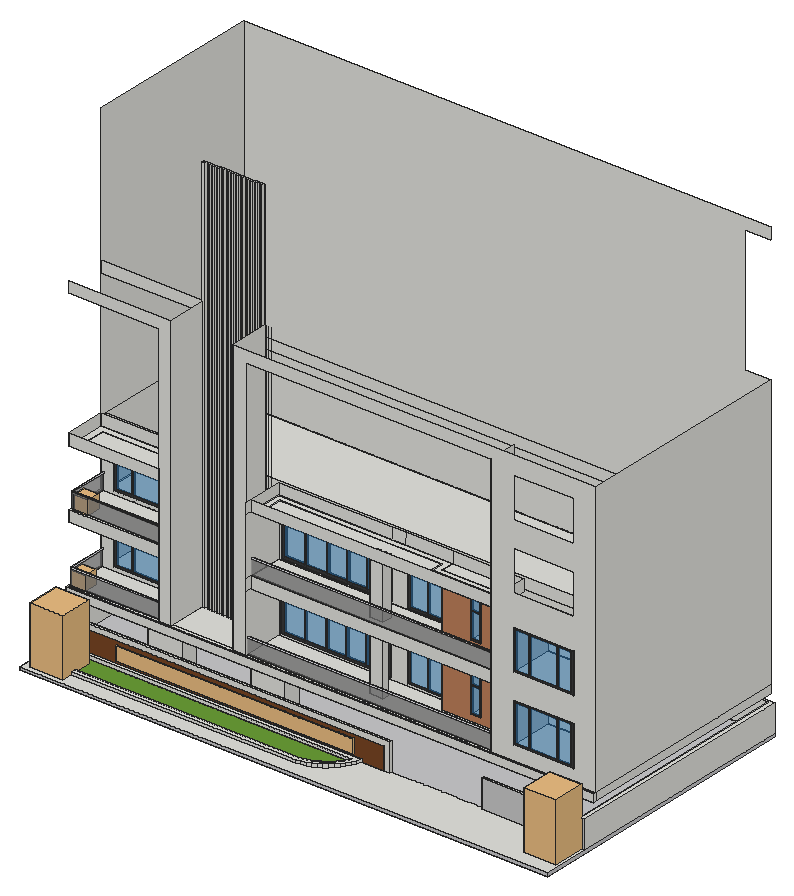
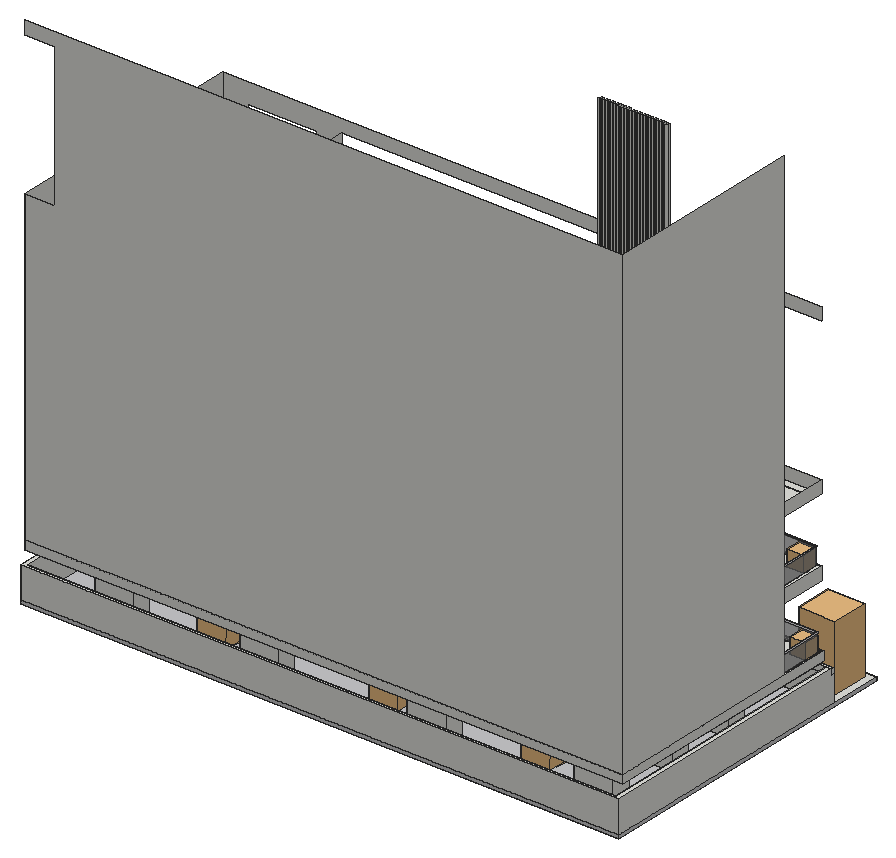
# SketchUp Ruby script. Lengths in inches.
U = 1.inch
M = Sketchup.active_model
def pt(a) = Geom::Point3d.new(a.map { |v| v * U })
def face(e, loops, mat)
  f = e.add_face(loops[0].map { |a| pt(a) })
  loops[1..].each { |l| e.add_face(l.map { |a| pt(a) }).erase! }
  f.material = f.back_material = mat if mat
  f
end
# faces: each face lists its corners as indices into pts; further lists are holes
def faces(e, pts, list, mat = nil) = list.each { |f| face(e, (f[0].is_a?(Array) ? f : [f]).map { |l| l.map { |i| pts[i] } }, mat) }
# xy, xz, yz: faces in a plane at the given z, y or x. An outline is a flat list of corners, or four numbers for a rectangle; further outlines are holes
def ring(l) = l.size == 4 ? [[l[0], l[1]], [l[2], l[1]], [l[2], l[3]], [l[0], l[3]]] : l.each_slice(2).to_a
def flat(e, list, mat, &to3) = list.each { |f| face(e, (f[0].is_a?(Array) ? f : [f]).map { |l| ring(l).map { |u, v| to3.(u, v) } }, mat) }
def xy(e, z, list, mat = nil) = flat(e, list, mat) { |x, y| [x, y, z] }
def xz(e, y, list, mat = nil) = flat(e, list, mat) { |x, z| [x, y, z] }
def yz(e, x, list, mat = nil) = flat(e, list, mat) { |y, z| [x, y, z] }
def lines(e, pts, list) = list.each { |a, b| e.add_line(pt(pts[a]), pt(pts[b])) }
# prism: a flat outline (further loops are holes) pulled along v
def prism(e, loops, v, mat = nil)
  f = face(e, loops, mat); d = Geom::Vector3d.new(v.map { |x| x * U })
  f.pushpull(f.normal.samedirection?(d) ? d.length : -d.length)
end
def box(e, o, s, mat = nil) = prism(e, [[o, [o[0] + s[0], o[1], o[2]], [o[0] + s[0], o[1] + s[1], o[2]], [o[0], o[1] + s[1], o[2]]]], [0, 0, s[2]], mat)
def at(x, y, z, deg = 0) = Geom::Transformation.translation(pt([x, y, z])) * Geom::Transformation.rotation(ORIGIN, Z_AXIS, deg.degrees)
def axes(o, x, y, z) = Geom::Transformation.new([*x, 0, *y, 0, *z, 0, *pt(o).to_a, 1])
def part(name) = M.definitions.add(name)
# library, detail: a bought-in or finely detailed component or shape, given as its bounding box
def library(name, o, s) = part(name).tap { |d| box(d.entities, o, s) }
def detail(e, o, s) = box(e.add_group.entities, o, s)
def put(e, d, t, mat = nil) = e.add_instance(d, t).tap { |i| i.material = mat if mat }
def group(e, t, mat = nil) = e.add_group.tap { |g| g.transformation = t; g.material = mat if mat }.entities
root = M.entities
M.materials.add("[Cladding Stucco White]").color = [200, 200, 200]
M.materials.add("[Color M00]").color = [255, 255, 255]
M.materials.add("[Color M07]").color = [58, 58, 58]
M.materials.add("[Grass Dark Green]").color = [106, 157, 55]
M.materials.add("[Metal Silver]").color = [234, 233, 238]
M.materials.add("[Polished Concrete New]").color = [200, 200, 203]
M.materials.add("[Translucent Glass Gray]").color = [40, 128, 199]
M.materials["[Translucent Glass Gray]"].alpha = 0.5
M.materials.add("[Translucent Glass Gray]1").color = [128, 128, 128]
M.materials["[Translucent Glass Gray]1"].alpha = 0.5
M.materials.add("[Wood Veneer 01]").color = [120, 70, 37]
M.materials.add("[Wood Veneer 02]").color = [190, 128, 91]
c1 = library("skp28\#1",[-2.51,-5.3125,0.36],[4.33,10.51,2.73])
c2 = part("ske164\#1")
put(c2.entities,c1,axes([101.27,98.68,1.14],[21.38,0,0],[0,21.38,0],[0,0,21.38]))
c3 = library("ske17D",[0,0,0],[82.9,31.14,82.9])
c4 = part("Sedan car")
put(c4.entities,c2,at(-47.7,14.91,-2.5))
put(c4.entities,c3,axes([87.34,31.1,0],[0,0.35842,0],[-0.35842,0,0],[0,0,0.35842]))
put(c4.entities,c3,axes([87.34,160.85,0],[0,0.35842,0],[-0.35842,0,0],[0,0,0.35842]))
put(c4.entities,c3,axes([5.18,190.5625,0],[0,-0.35842,0],[0.35842,0,0],[0,0,0.35842]))
put(c4.entities,c3,axes([5.43,60.8125,0],[0,-0.35842,0],[0.35842,0,0],[0,0,0.35842]))
c5 = part("Audi car")
put(c5.entities,c4,axes([116.24,65.71,-0.51],[0.88343,0,-0.01128],[0.00041,0.88291,0.03237],[0.01127,-0.03237,0.88283]))
c6 = library("trees",[-21.19,-21.7,-0.46],[44.22,41.02,72.81])
c7 = library("ROSELINE\#1",[1.48,0,0],[414.76,59.92,4])
c8 = library("plants",[-16.3,-15.81,0],[32.6,31.62,37.8])
c9 = part("Group\#3")
xy(c9.entities,0,[[0,0,103.1875,6]],"[Color M07]")
xy(c9.entities,6.75,[[6.75,0,49.1,6],[51.71,0,96.4375,6]],"[Color M07]")
xy(c9.entities,160.21,[[6.75,0,49.1,6],[51.71,0,96.4375,6]],"[Color M07]")
xy(c9.entities,166.96,[[0,0,103.1875,6]],"[Color M07]")
xz(c9.entities,0,[[[0,0,103.1875,166.96],[51.71,6.75,96.4375,160.21],[6.75,6.75,49.1,160.21]]],"[Color M07]")
xz(c9.entities,0,[[6.75,6.75,49.1,160.21],[51.71,6.75,96.4375,160.21]],"[Translucent Glass Gray]")
xz(c9.entities,6,[[[0,0,103.1875,166.96],[51.71,6.75,96.4375,160.21],[6.75,6.75,49.1,160.21]]],"[Color M07]")
yz(c9.entities,0,[[0,0,6,166.96]],"[Color M07]")
yz(c9.entities,6.75,[[0,6.75,6,160.21]],"[Color M07]")
yz(c9.entities,49.1,[[0,6.75,6,160.21]],"[Color M07]")
yz(c9.entities,51.71,[[0,6.75,6,160.21]],"[Color M07]")
yz(c9.entities,96.4375,[[0,6.75,6,160.21]],"[Color M07]")
yz(c9.entities,103.1875,[[0,0,6,166.96]],"[Color M07]")
c10 = part("Group\#2")
xy(c10.entities,0,[[0,0,266.875,6]],"[Color M07]")
xy(c10.entities,9.27,[[9.27,0,57.67,6],[61.37,0,109.48,6],[113.18,0,157.6,6],[161.3,0,205.85,6],[209.55,0,257.6,6]],"[Color M07]")
xy(c10.entities,155.66,[[9.27,0,57.67,6],[61.37,0,109.48,6],[113.18,0,157.6,6],[161.3,0,205.85,6],[209.55,0,257.6,6]],"[Color M07]")
xy(c10.entities,164.9375,[[0,0,266.875,6]],"[Color M07]")
xz(c10.entities,0,[[[0,0,266.875,164.9375],[9.27,9.27,57.67,155.66],[61.37,9.27,109.48,155.66],[209.55,9.27,257.6,155.66],[161.3,9.27,205.85,155.66],[113.18,9.27,157.6,155.66]]],"[Color M07]")
xz(c10.entities,0,[[9.27,9.27,57.67,155.66],[61.37,9.27,109.48,155.66],[113.18,9.27,157.6,155.66],[161.3,9.27,205.85,155.66],[209.55,9.27,257.6,155.66]],"[Translucent Glass Gray]")
xz(c10.entities,6,[[[0,0,266.875,164.9375],[9.27,9.27,57.67,155.66],[61.37,9.27,109.48,155.66],[209.55,9.27,257.6,155.66],[161.3,9.27,205.85,155.66],[113.18,9.27,157.6,155.66]]],"[Color M07]")
yz(c10.entities,0,[[0,0,6,164.9375]],"[Color M07]")
yz(c10.entities,9.27,[[0,9.27,6,155.66]],"[Color M07]")
yz(c10.entities,57.67,[[0,9.27,6,155.66]],"[Color M07]")
yz(c10.entities,61.37,[[0,9.27,6,155.66]],"[Color M07]")
yz(c10.entities,109.48,[[0,9.27,6,155.66]],"[Color M07]")
yz(c10.entities,113.18,[[0,9.27,6,155.66]],"[Color M07]")
yz(c10.entities,157.6,[[0,9.27,6,155.66]],"[Color M07]")
yz(c10.entities,161.3,[[0,9.27,6,155.66]],"[Color M07]")
yz(c10.entities,205.85,[[0,9.27,6,155.66]],"[Color M07]")
yz(c10.entities,209.55,[[0,9.27,6,155.66]],"[Color M07]")
yz(c10.entities,257.6,[[0,9.27,6,155.66]],"[Color M07]")
yz(c10.entities,266.875,[[0,0,6,164.9375]],"[Color M07]")
c11 = part("Group\#4")
xy(c11.entities,0,[[0,0,117.92,3.42]],"[Color M07]")
xy(c11.entities,5.06,[[5.06,0,29.89,3.42],[33.27,0,84.5,3.42],[87.88,0,112.86,3.42]],"[Color M07]")
xy(c11.entities,112.86,[[5.06,0,29.89,3.42],[33.27,0,84.5,3.42],[87.88,0,112.86,3.42]],"[Color M07]")
xy(c11.entities,117.92,[[0,0,117.92,3.42]],"[Color M07]")
xz(c11.entities,0,[[[0,0,117.92,117.92],[33.27,5.06,84.5,112.86],[87.88,5.06,112.86,112.86],[5.06,5.06,29.89,112.86]]],"[Color M07]")
xz(c11.entities,0,[[5.06,5.06,29.89,112.86],[33.27,5.06,84.5,112.86],[87.88,5.06,112.86,112.86]],"[Translucent Glass Gray]")
xz(c11.entities,3.42,[[[0,0,117.92,117.92],[33.27,5.06,84.5,112.86],[87.88,5.06,112.86,112.86],[5.06,5.06,29.89,112.86]]],"[Color M07]")
yz(c11.entities,0,[[0,0,3.42,117.92]],"[Color M07]")
yz(c11.entities,5.06,[[0,5.06,3.42,112.86]],"[Color M07]")
yz(c11.entities,29.89,[[0,5.06,3.42,112.86]],"[Color M07]")
yz(c11.entities,33.27,[[0,5.06,3.42,112.86]],"[Color M07]")
yz(c11.entities,84.5,[[0,5.06,3.42,112.86]],"[Color M07]")
yz(c11.entities,87.88,[[0,5.06,3.42,112.86]],"[Color M07]")
yz(c11.entities,112.86,[[0,5.06,3.42,112.86]],"[Color M07]")
yz(c11.entities,117.92,[[0,0,3.42,117.92]],"[Color M07]")
c12 = part("Group\#5")
xy(c12.entities,0,[[0,0,33.625,2.4375]],"[Color M07]")
xy(c12.entities,2.77,[[2.77,0,30.85,2.4375]],"[Color M07]")
xy(c12.entities,92.73,[[2.77,0,30.85,2.4375]],"[Color M07]")
xy(c12.entities,95.66,[[2.77,0,30.85,2.4375]],"[Color M07]")
xy(c12.entities,164.1,[[2.77,0,30.85,2.4375]],"[Color M07]")
xy(c12.entities,166.875,[[0,0,33.625,2.4375]],"[Color M07]")
xz(c12.entities,0,[[[0,0,33.625,166.875],[2.77,2.77,30.85,92.73],[2.77,95.66,30.85,164.1]]],"[Color M07]")
xz(c12.entities,0,[[2.77,2.77,30.85,92.73],[2.77,95.66,30.85,164.1]],"[Translucent Glass Gray]")
xz(c12.entities,2.4375,[[[0,0,33.625,166.875],[2.77,2.77,30.85,92.73],[2.77,95.66,30.85,164.1]]],"[Color M07]")
yz(c12.entities,0,[[0,0,2.4375,166.875]],"[Color M07]")
yz(c12.entities,2.77,[[0,2.77,2.4375,92.73],[0,95.66,2.4375,164.1]],"[Color M07]")
yz(c12.entities,30.85,[[0,2.77,2.4375,92.73],[0,95.66,2.4375,164.1]],"[Color M07]")
yz(c12.entities,33.625,[[0,0,2.4375,166.875]],"[Color M07]")
xy(root,0,[[0,0,1665.48,897.1]])
xy(root,9,[[0,0,1665.48,0,1665.48,149.5,1338.12,149.5,1338.12,157.51,1048.18,157.51,1048.18,149.5,958.59,149.5,953.98,136.02,948.06,123.06,940.88,110.75,932.53,99.2,923.07,88.54,912.61,78.87,901.25,70.28,889.09,62.85,876.25,56.66,862.87,51.77,849.07,48.23,834.98,46.0625,84.59,46.0625,84.59,149.5,0,149.5],[[84.59,46.0625,84.59,149.5,958.59,149.5,953.98,136.02,948.06,123.06,940.88,110.75,932.53,99.2,923.07,88.54,912.61,78.87,901.25,70.28,889.09,62.85,876.25,56.66,862.87,51.77,849.07,48.23,834.98,46.0625],[97.76,59.23,833.98,59.23,846.42,61.14,858.96,64.36,871.12,68.8,882.78,74.43,893.83,81.17,904.15,88.98,913.66,97.77,922.25,107.45,929.84,117.9375,936.35,129.12,939.65,136.33,97.76,136.33]],[0,149.5,0,897.1,1665.48,897.1,1665.48,149.5,1338.12,149.5,1338.12,157.51,1651.6,157.51,1651.6,889.09,13.88,889.09,13.88,157.51,1030.62,157.51,1030.62,149.5],[1030.62,149.5,1048.18,157.51],[221.91,227.7,330.82,281.1],
  [546.04,227.7,654.95,281.1],[81.13,358.18,190.04,411.58],[1412.71,362.14,1521.62,415.54],[81.13,553.59,190.04,606.99],[1412.71,567.51,1521.62,620.91],
  [81.13,760.57,190.04,813.97],[542.67,764.37,651.58,817.77],[1009.74,764.37,1118.65,817.77],[1412.71,764.37,1521.62,817.77]])
xy(root,9,[[97.76,59.23,833.98,59.23,846.42,61.14,858.96,64.36,871.12,68.8,882.78,74.43,893.83,81.17,904.15,88.98,913.66,97.77,922.25,107.45,929.84,117.9375,936.35,129.12,939.65,136.33,97.76,136.33]],"[Grass Dark Green]")
xy(root,9,[[[13.88,157.51,1651.6,889.09],[221.91,227.7,330.82,281.1],[546.04,227.7,654.95,281.1],[81.13,760.57,190.04,813.97],[81.13,553.59,190.04,606.99],[81.13,358.18,190.04,411.58],[1009.74,764.37,1118.65,817.77],[1412.71,764.37,1521.62,817.77],[1412.71,567.51,1521.62,620.91],[1412.71,362.14,1521.62,415.54],[542.67,764.37,651.58,817.77]]],"[Polished Concrete New]")
xy(root,17.8125,[[[84.59,46.0625,834.98,46.0625,849.07,48.23,862.87,51.77,876.25,56.66,889.09,62.85,901.25,70.28,912.61,78.87,923.07,88.54,932.53,99.2,940.88,110.75,948.06,123.06,953.98,136.02,958.59,149.5,84.59,149.5],[97.76,59.23,97.76,136.33,939.65,136.33,936.35,129.12,929.84,117.9375,922.25,107.45,913.66,97.77,904.15,88.98,893.83,81.17,882.78,74.43,871.12,68.8,858.96,64.36,846.42,61.14,833.98,59.23]]])
xy(root,98.25,[[0,149.5,1048.18,157.51],[1338.12,149.5,1665.48,149.5,1665.48,897.1,0,897.1,0,157.51,13.88,157.51,13.88,889.09,1651.6,889.09,1651.6,157.51,1338.12,157.51]])
xy(root,129,[[0,182.16,1665.48,191.16]])
xy(root,129,[[[0,191.16,1665.48,882.45],[221.91,227.7,330.82,281.1],[546.04,227.7,654.95,281.1],[1009.74,764.37,1118.65,817.77],[81.13,760.57,190.04,813.97],[1412.71,362.14,1521.62,415.54],[1412.71,567.51,1521.62,620.91],[542.67,764.37,651.58,817.77],[81.13,553.59,190.04,606.99],[81.13,358.18,190.04,411.58],[1412.71,764.37,1521.62,817.77]],[221.91,227.7,330.82,281.1],[546.04,227.7,654.95,281.1],[81.13,358.18,190.04,411.58],[1412.71,362.14,1521.62,415.54],
  [81.13,553.59,190.04,606.99],[1412.71,567.51,1521.62,620.91],[81.13,760.57,190.04,813.97],[542.67,764.37,651.58,817.77],[1009.74,764.37,1118.65,817.77],
  [1412.71,764.37,1521.62,817.77]],"[Color M00]")
xy(root,153,[[0,182.16,1665.48,182.16,1665.48,187.35,4.5625,187.35,4.5625,320.73,0,320.73],[4.5625,187.35,1665.48,187.35,1665.48,191.16,1334.26,191.16,1334.26,195.98,559.99,195.98,559.99,191.16,518.01,191.16,518.01,196.41,324.77,196.41,324.77,191.16,284.54,191.16,284.54,196.41,4.5625,196.41],[518.01,191.16,518.01,320.73,0,320.73,0,882.45,1561.7,882.45,1561.7,873.45,9.75,873.45,9.75,328.54,1561.7,328.54,1561.7,191.16,1334.26,191.16,1334.26,280.1,1109.39,280.1,1109.39,320.73,559.99,320.73,559.99,191.16],[284.54,191.16,324.77,320.73],[1561.7,191.16,1561.7,328.54,1655.73,328.54,1655.73,873.45,1561.7,873.45,1561.7,882.45,1665.48,882.45,1665.48,191.16],
  [559.99,195.98,1334.26,197.98],[4.5625,196.41,284.54,198.73],[[559.99,197.98,1334.26,197.98,1334.26,280.1,1109.39,280.1,1109.39,320.73,559.99,320.73],[917.6,233.32,960.55,250.32]],[4.5625,198.73,6.5625,320.73],[6.5625,198.73,284.54,320.73],
  [324.77,198.73,518.01,198.73,518.01,320.73,514,320.73,514,313.48,506.5,313.48,506.5,320.73,499,320.73,499,313.48,491.5,313.48,491.5,320.73,484,320.73,484,313.48,476.5,313.48,476.5,320.73,469,320.73,469,313.48,461.5,313.48,461.5,320.73,454,320.73,454,313.48,446.5,313.48,446.5,320.73,439,320.73,439,313.48,431.5,313.48,431.5,320.73,424,320.73,424,313.48,416.5,313.48,416.5,320.73,409,320.73,409,313.48,401.5,313.48,401.5,320.73,394,320.73,394,313.48,386.5,313.48,386.5,320.73,379,320.73,379,313.48,371.5,313.48,371.5,320.73,364,320.73,364,313.48,356.5,313.48,356.5,320.73,349,320.73,349,313.48,341.5,313.48,341.5,320.73,334,320.73,334,313.48,324.77,313.48],[917.6,233.32,960.55,250.32],[324.77,313.48,334,320.73],[341.5,313.48,349,320.73],[356.5,313.48,364,320.73],
  [371.5,313.48,379,320.73],[386.5,313.48,394,320.73],[401.5,313.48,409,320.73],[416.5,313.48,424,320.73],[431.5,313.48,439,320.73],
  [446.5,313.48,454,320.73],[461.5,313.48,469,320.73],[476.5,313.48,484,320.73],[491.5,313.48,499,320.73],[506.5,313.48,514,320.73],
  [9.75,328.54,1561.7,873.45],[1561.7,328.54,1655.73,873.45]])
xy(root,157.44,[[967.92,320.73,1101.04,328.54]])
xy(root,157.96,[[566.1875,320.73,914.8125,328.54]])
xy(root,163.04,[[40.45,320.73,260.7,328.54]])
xy(root,172.9,[[1200.375,280.1,1230.875,328.54]])
xy(root,196.42,[[1405.04,191.16,1595.91,328.54]])
xy(root,201,[[559.99,195.98,1334.26,197.98],[4.5625,196.41,4.5625,320.73,6.5625,320.73,6.5625,198.73,284.54,198.73,284.54,196.41]],"[Metal Silver]")
xy(root,205,[[559.99,195.98,1334.26,197.98],[4.5625,196.41,284.54,196.41,284.54,198.73,6.5625,198.73,6.5625,320.73,4.5625,320.73]],"[Metal Silver]")
xy(root,302.7,[[566.1875,320.73,914.8125,328.54],[967.92,320.73,1101.04,328.54]])
xy(root,316.92,[[40.45,320.73,260.7,328.54]])
xy(root,319.08,[[1200.375,280.1,1230.875,328.54]])
xy(root,324.73,[[1405.04,191.16,1595.91,328.54]])
xy(root,325,[[[578.25,228.93,578.25,302.47,1091.125,302.47,1091.125,261.84,1316,261.84,1316,228.93],[917.6,233.32,960.55,250.32]]])
xy(root,328,[[17.43,208.59,267.11,303.3]])
xy(root,333,[[[0,191.16,284.54,320.73],[17.43,208.59,267.11,303.3]],[17.43,208.59,267.11,303.3],[[559.99,210.66,559.99,320.73,1109.39,320.73,1109.39,280.1,1334.26,280.1,1334.26,210.66],[578.25,228.93,1316,228.93,1316,261.84,1091.125,261.84,1091.125,302.47,578.25,302.47]],[[578.25,228.93,1316,228.93,1316,261.84,1091.125,261.84,1091.125,302.47,578.25,302.47],[917.6,233.32,960.55,250.32]],[917.6,233.32,960.55,250.32],
  [1109.39,280.1,1334.26,320.73]])
xy(root,369,[[0,191.16,284.54,191.16,284.54,197.23,6.5625,197.23,6.5625,320.73,0,320.73],[6.5625,197.23,6.5625,320.73,8.5625,320.73,8.5625,199.23,284.54,199.23,284.54,197.23],[8.5625,199.23,284.54,320.73],[559.99,210.66,1334.26,212.66],[559.99,212.66,1334.26,214.66],
  [[559.99,214.66,1334.26,214.66,1334.26,280.1,1109.39,280.1,1109.39,320.73,559.99,320.73],[917.6,233.32,960.55,264.07]],[917.6,233.32,960.55,264.07],[1109.39,280.1,1334.26,320.73],[9.75,328.54,1561.7,873.45]])
xy(root,371.75,[[967.92,320.73,1101.04,328.54]])
xy(root,373.36,[[568.97,320.73,917.6,328.54]])
xy(root,379.67,[[40.45,320.73,260.7,328.54]])
xy(root,383.4,[[1200.375,280.1,1230.875,328.54]])
xy(root,402.17,[[1405.04,191.16,1595.91,328.54]])
xy(root,417,[[6.5625,197.23,6.5625,320.73,8.5625,320.73,8.5625,199.23,284.54,199.23,284.54,197.23],[559.99,212.66,1334.26,214.66]],"[Metal Silver]")
xy(root,421,[[6.5625,197.23,284.54,197.23,284.54,199.23,8.5625,199.23,8.5625,320.73,6.5625,320.73],[559.99,212.66,1334.26,214.66]],"[Metal Silver]")
xy(root,522.07,[[568.97,320.73,917.6,328.54],[967.92,320.73,1101.04,328.54]])
xy(root,529.58,[[1200.375,280.1,1230.875,328.54]])
xy(root,530.48,[[1405.04,191.16,1595.91,328.54]])
xy(root,533.54,[[40.45,320.73,260.7,328.54]])
xy(root,541,[[[578.25,228.93,578.25,302.47,1091.125,302.47,1091.125,261.84,1316,261.84,1316,228.93],[917.6,233.32,960.55,264.07]]])
xy(root,544,[[21.22,212.38,263.32,299.51]])
xy(root,549,[[[0,191.16,284.54,320.73],[21.22,212.38,263.32,299.51]],[[559.99,210.66,559.99,320.73,1109.39,320.73,1109.39,280.1,1334.26,280.1,1334.26,210.66],[578.25,228.93,1316,228.93,1316,261.84,1091.125,261.84,1091.125,302.47,578.25,302.47]],[21.22,212.38,263.32,299.51],[[578.25,228.93,1316,228.93,1316,261.84,1091.125,261.84,1091.125,302.47,578.25,302.47],[917.6,233.32,960.55,264.07]],[1109.39,280.1,1334.26,320.73]])
xz(root,0,[[0,0,1665.48,9]],"[Polished Concrete New]")
xz(root,46.0625,[[84.59,9,834.98,17.8125]])
xz(root,59.23,[[97.76,9,833.98,17.8125]])
xz(root,136.33,[[97.76,9,939.65,17.8125]])
xz(root,149.5,[[0,9,27.05,9,27.05,81,1030.62,81,1030.62,9,1048.18,9,1048.18,98.25,0,98.25],[84.59,9,958.59,17.8125]])
xz(root,149.5,[[1338.12,9,1665.48,98.25]],"[Cladding Stucco White]")
xz(root,149.5,[[27.05,9,84.59,9,84.59,17.8125,958.59,17.8125,958.59,9,1030.62,9,1030.62,81,27.05,81]],"[Wood Veneer 01]")
xz(root,157.51,[[1030.62,9,1030.62,81,13.88,81,13.88,98.25,1048.18,98.25,1048.18,9],[13.88,9,1030.62,81],[1338.12,9,1651.6,98.25]])
xz(root,182.16,[[0,129,1665.48,153]])
xz(root,191.16,[[284.54,153,324.77,153,324.77,1017,0,1017,0,981,284.54,981],[[518.01,153,559.99,153,559.99,981,1334.26,981,1334.26,153,1665.48,153,1665.48,1017,518.01,1017],[1405.04,832.73,1595.91,961.04],[1405.04,625.17,1595.91,753.48],[1405.04,196.42,1595.91,324.73],[1405.04,402.17,1595.91,530.48]],[0,333,284.54,369],[0,549,284.54,585]])
xz(root,195.98,[[559.99,201,1334.26,205]],"[Metal Silver]")
xz(root,195.98,[[559.99,153,1334.26,201]],"[Translucent Glass Gray]1")
xz(root,196.41,[[4.5625,201,284.54,205]],"[Metal Silver]")
xz(root,196.41,[[4.5625,153,284.54,201]],"[Translucent Glass Gray]1")
xz(root,197.23,[[6.5625,417,284.54,421]],"[Metal Silver]")
xz(root,197.23,[[6.5625,369,284.54,417]],"[Translucent Glass Gray]1")
xz(root,197.98,[[559.99,201,1334.26,205]],"[Metal Silver]")
xz(root,197.98,[[559.99,153,1334.26,201]],"[Translucent Glass Gray]1")
xz(root,198.73,[[6.5625,201,284.54,205]],"[Metal Silver]")
xz(root,198.73,[[6.5625,153,284.54,201]],"[Translucent Glass Gray]1")
xz(root,199.23,[[8.5625,417,284.54,421]],"[Metal Silver]")
xz(root,199.23,[[8.5625,369,284.54,417]],"[Translucent Glass Gray]1")
xz(root,208.59,[[17.43,328,267.11,333]])
xz(root,210.66,[[559.99,333,1334.26,369],[559.99,549,1334.26,585]])
xz(root,212.38,[[21.22,544,263.32,549]])
xz(root,212.66,[[559.99,417,1334.26,421]],"[Metal Silver]")
xz(root,212.66,[[559.99,369,1334.26,417]],"[Translucent Glass Gray]1")
xz(root,214.66,[[559.99,417,1334.26,421]],"[Metal Silver]")
xz(root,214.66,[[559.99,369,1334.26,417]],"[Translucent Glass Gray]1")
xz(root,227.7,[[221.91,9,330.82,129],[546.04,9,654.95,129]])
xz(root,228.93,[[578.25,325,1316,333],[578.25,541,1316,549]])
xz(root,233.32,[[917.6,153,960.55,325],[917.6,325,960.55,333],[917.6,369,960.55,541],[917.6,541,960.55,549]])
xz(root,250.32,[[917.6,153,960.55,325],[917.6,325,960.55,333]])
xz(root,261.84,[[1091.125,325,1316,333],[1091.125,541,1316,549]])
xz(root,264.07,[[917.6,369,960.55,541],[917.6,541,960.55,549]])
xz(root,280.1,[[[1109.39,153,1334.26,333],[1200.375,172.9,1230.875,319.08]],[[1109.39,369,1334.26,549],[1200.375,383.4,1230.875,529.58]]],"[Wood Veneer 02]")
xz(root,281.1,[[221.91,9,330.82,129],[546.04,9,654.95,129]])
xz(root,299.51,[[21.22,544,263.32,549]])
xz(root,302.47,[[578.25,325,917.6,333],[917.6,325,960.55,333],[960.55,325,1091.125,333],[578.25,541,917.6,549],[917.6,541,960.55,549],
  [960.55,541,1091.125,549]])
xz(root,303.3,[[17.43,328,267.11,333]])
xz(root,313.48,[[324.77,153,334,1413],[341.5,153,349,1413],[356.5,153,364,1413],[371.5,153,379,1413],[386.5,153,394,1413],
  [401.5,153,409,1413],[416.5,153,424,1413],[431.5,153,439,1413],[446.5,153,454,1413],[461.5,153,469,1413],
  [476.5,153,484,1413],[491.5,153,499,1413],[506.5,153,514,1413]])
xz(root,320.73,[[284.54,153,284.54,981,0,981,0,1017,324.77,1017,324.77,153],[[0,153,4.5625,153,4.5625,205,6.5625,205,6.5625,153,284.54,153,284.54,333,0,333],[40.45,163.04,260.7,316.92]],[4.5625,153,6.5625,201],[324.77,153,334,1413],[334,153,341.5,1413],
  [341.5,153,349,1413],[349,153,356.5,1413],[356.5,153,364,1413],[364,153,371.5,1413],[371.5,153,379,1413],
  [379,153,386.5,1413],[386.5,153,394,1413],[394,153,401.5,1413],[401.5,153,409,1413],[409,153,416.5,1413],
  [416.5,153,424,1413],[424,153,431.5,1413],[431.5,153,439,1413],[439,153,446.5,1413],[446.5,153,454,1413],
  [454,153,461.5,1413],[461.5,153,469,1413],[469,153,476.5,1413],[476.5,153,484,1413],[484,153,491.5,1413],
  [491.5,153,499,1413],[499,153,506.5,1413],[506.5,153,514,1413],[514,153,518.01,1413],[[559.99,153,1109.39,333],[566.1875,157.96,914.8125,302.7],[967.92,157.44,1101.04,302.7]],
  [0,333,284.54,369],[559.99,333,917.6,369],[917.6,333,960.55,369],[960.55,333,1109.39,369],[1109.39,333,1334.26,369],
  [[0,369,6.5625,369,6.5625,421,8.5625,421,8.5625,369,284.54,369,284.54,549,0,549],[40.45,379.67,260.7,533.54]],[6.5625,369,8.5625,417],[[559.99,369,1109.39,549],[568.97,373.36,917.6,522.07],[967.92,371.75,1101.04,522.07]],[0,549,284.54,585],[559.99,549,917.6,585],
  [917.6,549,960.55,585],[960.55,549,1109.39,585],[1109.39,549,1334.26,585]])
xz(root,320.73,[[4.5625,201,6.5625,205],[6.5625,417,8.5625,421]],"[Metal Silver]")
xz(root,328.54,[[[9.75,153,1655.73,333],[566.1875,157.96,914.8125,302.7],[40.45,163.04,260.7,316.92],[1405.04,196.42,1595.91,324.73],[967.92,157.44,1101.04,302.7],[1200.375,172.9,1230.875,319.08]],[9.75,333,1655.73,369],[[9.75,369,1655.73,549],[568.97,373.36,917.6,522.07],[40.45,379.67,260.7,533.54],[1405.04,402.17,1595.91,530.48],[967.92,371.75,1101.04,522.07],[1200.375,383.4,1230.875,529.58]],[9.75,549,1655.73,585]])
xz(root,358.18,[[81.13,9,190.04,129]])
xz(root,362.14,[[1412.71,9,1521.62,129]])
xz(root,411.58,[[81.13,9,190.04,129]])
xz(root,415.54,[[1412.71,9,1521.62,129]])
xz(root,553.59,[[81.13,9,190.04,129]])
xz(root,567.51,[[1412.71,9,1521.62,129]])
xz(root,606.99,[[81.13,9,190.04,129]])
xz(root,620.91,[[1412.71,9,1521.62,129]])
xz(root,760.57,[[81.13,9,190.04,129]])
xz(root,764.37,[[542.67,9,651.58,129],[1009.74,9,1118.65,129],[1412.71,9,1521.62,129]])
xz(root,813.97,[[81.13,9,190.04,129]])
xz(root,817.77,[[542.67,9,651.58,129],[1009.74,9,1118.65,129],[1412.71,9,1521.62,129]])
xz(root,873.45,[[9.75,153,1655.73,333],[9.75,333,1655.73,369],[9.75,369,1655.73,549],[9.75,549,1655.73,585]])
xz(root,882.45,[[0,129,1665.48,153],[0,153,0,1449,1665.48,1449,1665.48,1413,1581.35,1413,1581.35,1017,1665.48,1017,1665.48,153]])
xz(root,889.09,[[13.88,9,1651.6,98.25]])
xz(root,897.1,[[0,9,1665.48,98.25]])
xz(root,897.1,[[0,0,1665.48,9]],"[Polished Concrete New]")
yz(root,0,[[149.5,9,149.5,81,157.51,81,157.51,98.25,897.1,98.25,897.1,9],[149.5,81,157.51,98.25],[182.16,129,882.45,153],[320.73,153,882.45,1449],[191.16,333,320.73,369],
  [191.16,549,320.73,585]])
yz(root,0,[[0,0,897.1,9]],"[Polished Concrete New]")
yz(root,4.5625,[[196.41,201,320.73,205]],"[Metal Silver]")
yz(root,4.5625,[[196.41,153,320.73,201]],"[Translucent Glass Gray]1")
yz(root,6.5625,[[198.73,201,320.73,205],[197.23,417,320.73,421]],"[Metal Silver]")
yz(root,6.5625,[[198.73,153,320.73,201],[197.23,369,320.73,417]],"[Translucent Glass Gray]1")
yz(root,8.5625,[[199.23,417,320.73,421]],"[Metal Silver]")
yz(root,8.5625,[[199.23,369,320.73,417]],"[Translucent Glass Gray]1")
yz(root,9.75,[[328.54,153,873.45,369],[328.54,369,873.45,585]])
yz(root,13.88,[[157.51,9,889.09,98.25]])
yz(root,17.43,[[208.59,328,303.3,333]])
yz(root,21.22,[[212.38,544,299.51,549]])
yz(root,40.45,[[320.73,163.04,328.54,316.92],[320.73,379.67,328.54,533.54]])
yz(root,81.13,[[358.18,9,411.58,129],[553.59,9,606.99,129],[760.57,9,813.97,129]])
yz(root,84.59,[[46.0625,9,149.5,17.8125]])
yz(root,97.76,[[59.23,9,136.33,17.8125]])
yz(root,190.04,[[358.18,9,411.58,129],[553.59,9,606.99,129],[760.57,9,813.97,129]])
yz(root,221.91,[[227.7,9,281.1,129]])
yz(root,260.7,[[320.73,163.04,328.54,316.92],[320.73,379.67,328.54,533.54]])
yz(root,263.32,[[212.38,544,299.51,549]])
yz(root,267.11,[[208.59,328,303.3,333]])
yz(root,284.54,[[191.16,153,191.16,333,320.73,333,320.73,153,198.73,153,198.73,205,196.41,205,196.41,153],[196.41,153,198.73,201],[191.16,333,320.73,369],[191.16,369,191.16,549,320.73,549,320.73,369,199.23,369,199.23,421,197.23,421,197.23,369],[197.23,369,199.23,417],
  [191.16,549,320.73,585]])
yz(root,284.54,[[196.41,201,198.73,205],[197.23,417,199.23,421]],"[Metal Silver]")
yz(root,324.77,[[191.16,153,313.48,1017],[313.48,153,320.73,333],[313.48,333,320.73,369],[313.48,369,320.73,549],[313.48,549,320.73,585]])
yz(root,330.82,[[227.7,9,281.1,129]])
yz(root,334,[[313.48,153,320.73,1413]])
yz(root,341.5,[[313.48,153,320.73,1413]])
yz(root,349,[[313.48,153,320.73,1413]])
yz(root,356.5,[[313.48,153,320.73,1413]])
yz(root,364,[[313.48,153,320.73,1413]])
yz(root,371.5,[[313.48,153,320.73,1413]])
yz(root,379,[[313.48,153,320.73,1413]])
yz(root,386.5,[[313.48,153,320.73,1413]])
yz(root,394,[[313.48,153,320.73,1413]])
yz(root,401.5,[[313.48,153,320.73,1413]])
yz(root,409,[[313.48,153,320.73,1413]])
yz(root,416.5,[[313.48,153,320.73,1413]])
yz(root,424,[[313.48,153,320.73,1413]])
yz(root,431.5,[[313.48,153,320.73,1413]])
yz(root,439,[[313.48,153,320.73,1413]])
yz(root,446.5,[[313.48,153,320.73,1413]])
yz(root,454,[[313.48,153,320.73,1413]])
yz(root,461.5,[[313.48,153,320.73,1413]])
yz(root,469,[[313.48,153,320.73,1413]])
yz(root,476.5,[[313.48,153,320.73,1413]])
yz(root,484,[[313.48,153,320.73,1413]])
yz(root,491.5,[[313.48,153,320.73,1413]])
yz(root,499,[[313.48,153,320.73,1413]])
yz(root,506.5,[[313.48,153,320.73,1413]])
yz(root,514,[[313.48,153,320.73,1413]])
yz(root,518.01,[[191.16,153,320.73,1017]])
yz(root,542.67,[[764.37,9,817.77,129]])
yz(root,546.04,[[227.7,9,281.1,129]])
yz(root,559.99,[[191.16,153,195.98,153,195.98,205,197.98,205,197.98,153,320.73,153,320.73,333,191.16,333],[195.98,153,197.98,201],[191.16,333,210.66,369],[210.66,333,320.73,369],[191.16,369,212.66,369,212.66,421,214.66,421,214.66,369,320.73,369,320.73,549,191.16,549],
  [212.66,369,214.66,417],[191.16,549,210.66,585],[210.66,549,320.73,585]])
yz(root,559.99,[[195.98,201,197.98,205],[212.66,417,214.66,421]],"[Metal Silver]")
yz(root,566.1875,[[320.73,157.96,328.54,302.7]])
yz(root,568.97,[[320.73,373.36,328.54,522.07]])
yz(root,578.25,[[228.93,325,302.47,333],[228.93,541,302.47,549]])
yz(root,651.58,[[764.37,9,817.77,129]])
yz(root,654.95,[[227.7,9,281.1,129]])
yz(root,914.8125,[[320.73,157.96,328.54,302.7]])
yz(root,917.6,[[233.32,153,250.32,325],[233.32,325,250.32,333],[233.32,369,264.07,541],[320.73,373.36,328.54,522.07],[233.32,541,264.07,549]])
yz(root,960.55,[[233.32,153,250.32,325],[233.32,325,250.32,333],[233.32,369,264.07,541],[233.32,541,264.07,549]])
yz(root,967.92,[[320.73,157.44,328.54,302.7],[320.73,371.75,328.54,522.07]])
yz(root,1009.74,[[764.37,9,817.77,129]])
yz(root,1030.62,[[149.5,9,157.51,81]])
yz(root,1048.18,[[149.5,9,157.51,98.25]])
yz(root,1091.125,[[261.84,325,302.47,333],[261.84,541,302.47,549]])
yz(root,1101.04,[[320.73,157.44,328.54,302.7],[320.73,371.75,328.54,522.07]])
yz(root,1109.39,[[280.1,153,320.73,333],[280.1,369,320.73,549]],"[Wood Veneer 02]")
yz(root,1118.65,[[764.37,9,817.77,129]])
yz(root,1200.375,[[280.1,172.9,328.54,319.08],[280.1,383.4,328.54,529.58]])
yz(root,1230.875,[[280.1,172.9,328.54,319.08],[280.1,383.4,328.54,529.58]])
yz(root,1316,[[228.93,325,261.84,333],[228.93,541,261.84,549]])
yz(root,1334.26,[[191.16,153,191.16,981,280.1,981,280.1,801,215.16,801,215.16,853,213.16,853,213.16,801,210.66,801,210.66,765,280.1,765,280.1,585,215.98,585,215.98,637,213.98,637,213.98,585,210.66,585,210.66,549,280.1,549,280.1,369,214.66,369,214.66,421,212.66,421,212.66,369,210.66,369,210.66,333,280.1,333,280.1,153,197.98,153,197.98,205,195.98,205,195.98,153],[195.98,153,197.98,201],[210.66,333,320.73,369],[212.66,369,214.66,417],[210.66,549,320.73,585]])
yz(root,1334.26,[[195.98,201,197.98,205],[212.66,417,214.66,421]],"[Metal Silver]")
yz(root,1338.12,[[149.5,9,157.51,98.25]])
yz(root,1405.04,[[191.16,196.42,328.54,324.73],[191.16,402.17,328.54,530.48]])
yz(root,1412.71,[[362.14,9,415.54,129],[567.51,9,620.91,129],[764.37,9,817.77,129]])
yz(root,1521.62,[[362.14,9,415.54,129],[567.51,9,620.91,129],[764.37,9,817.77,129]])
yz(root,1595.91,[[191.16,196.42,328.54,324.73],[191.16,402.17,328.54,530.48]])
yz(root,1651.6,[[157.51,9,889.09,98.25]])
yz(root,1665.48,[[149.5,9,897.1,98.25],[182.16,129,191.16,153],[191.16,129,882.45,153],[191.16,153,882.45,1017]])
yz(root,1665.48,[[0,0,897.1,9]],"[Polished Concrete New]")
p = [[834.98,46.0625,9],[849.07,48.23,9],[849.07,48.23,17.8125],[834.98,46.0625,17.8125],[862.87,51.77,9],[862.87,51.77,17.8125],
  [876.25,56.66,9],[876.25,56.66,17.8125],[889.09,62.85,9],[889.09,62.85,17.8125],[846.42,61.14,9],[833.98,59.23,9],
  [833.98,59.23,17.8125],[846.42,61.14,17.8125],[858.96,64.36,9],[858.96,64.36,17.8125],[901.25,70.28,9],[901.25,70.28,17.8125],
  [871.12,68.8,9],[871.12,68.8,17.8125],[882.78,74.43,9],[882.78,74.43,17.8125],[912.61,78.87,9],[912.61,78.87,17.8125],
  [893.83,81.17,9],[893.83,81.17,17.8125],[923.07,88.54,9],[923.07,88.54,17.8125],[904.15,88.98,9],[904.15,88.98,17.8125],
  [932.53,99.2,9],[932.53,99.2,17.8125],[913.66,97.77,9],[913.66,97.77,17.8125],[922.25,107.45,9],[922.25,107.45,17.8125],
  [940.88,110.75,9],[940.88,110.75,17.8125],[929.84,117.9375,9],[929.84,117.9375,17.8125],[948.06,123.06,9],[948.06,123.06,17.8125],
  [936.35,129.12,9],[936.35,129.12,17.8125],[953.98,136.02,9],[953.98,136.02,17.8125],[939.65,136.33,9],[939.65,136.33,17.8125],
  [958.59,149.5,9],[958.59,149.5,17.8125],[521.5,320.73,1017],[521.5,320.73,153],[529,320.73,1017],[529,320.73,153],
  [536.5,320.73,1017],[536.5,320.73,153]]
faces(root,p,[[0,1,2,3],[1,4,5,2],[4,6,7,5],[6,8,9,7],[10,11,12,13],[14,10,13,15],[8,16,17,9],[18,14,15,19],
  [20,18,19,21],[16,22,23,17],[24,20,21,25],[22,26,27,23],[28,24,25,29],[26,30,31,27],[32,28,29,33],[34,32,33,35],
  [30,36,37,31],[38,34,35,39],[36,40,41,37],[42,38,39,43],[40,44,45,41],[46,42,43,47],[44,48,49,45]])
lines(root,p,[[50,51],[52,53],[54,55]])
put(root,c5,at(1142.3,288.4375,9))
put(root,c6,axes([70.17,67.65,9.69],[2.3,0,0],[0,2.5,0],[0,0,2.5]))
put(root,c5,at(587.48,521.9,10.55))
put(root,c5,at(1049.06,541.76,10.55))
put(root,c5,at(810.82,324.43,10.55))
put(root,c5,at(162.86,521.9,10.55))
put(root,c5,at(292.62,288.54,10.55))
put(root,c6,axes([1601.08,101.19,10.14],[2.3,0,0],[0,2.5,0],[0,0,2.5]))
put(root,c7,axes([184.37,149.5,25.18],[1.8,0,0],[0,0,0.73],[0,-1,0]))
put(root,c8,axes([27.05,217.28,153],[1.38,0,0],[0,1.32,0],[0,0,1.15]))
put(root,c9,axes([967.33,320.96,157.44],[1.2958,0,0],[0,0.50741,0],[0,0,0.87003]))
put(root,c10,axes([566.1875,320.73,157.96],[1.30633,0,0],[0,0.83,0],[0,0,0.87128]))
put(root,c11,axes([40.45,320.73,163.04],[1.86781,0,0],[0,1,0],[0,0,1.30492]))
put(root,c12,axes([1200.375,279.23,172.9],[0.90706,0,0],[0,2.4,0],[0,0,0.87603]))
put(root,c11,axes([1405.04,191.16,196.42],[1.6187,0,0],[0,1,0],[0,0,1.08814]))
put(root,c8,axes([34.4,218.09,369],[1.38,0,0],[0,1.32,0],[0,0,1.15]))
put(root,c9,axes([967.92,320.73,371.75],[1.29013,0,0],[0,0.5456,0],[0,0,0.90029]))
put(root,c10,axes([568.97,320.73,373.36],[1.30633,0,0],[0,0.83,0],[0,0,0.90159]))
put(root,c11,axes([40.45,320.73,379.67],[1.86781,0,0],[0,1,0],[0,0,1.30492]))
put(root,c12,axes([1200.375,279.23,383.4],[0.90706,0,0],[0,2.4,0],[0,0,0.87603]))
put(root,c11,axes([1405.04,191.16,402.17],[1.6187,0,0],[0,1,0],[0,0,1.08814]))
